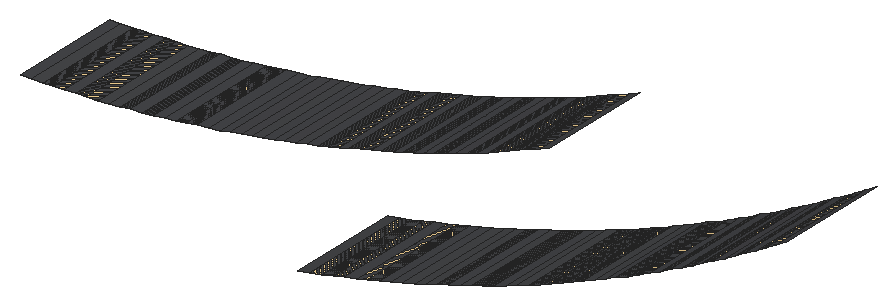
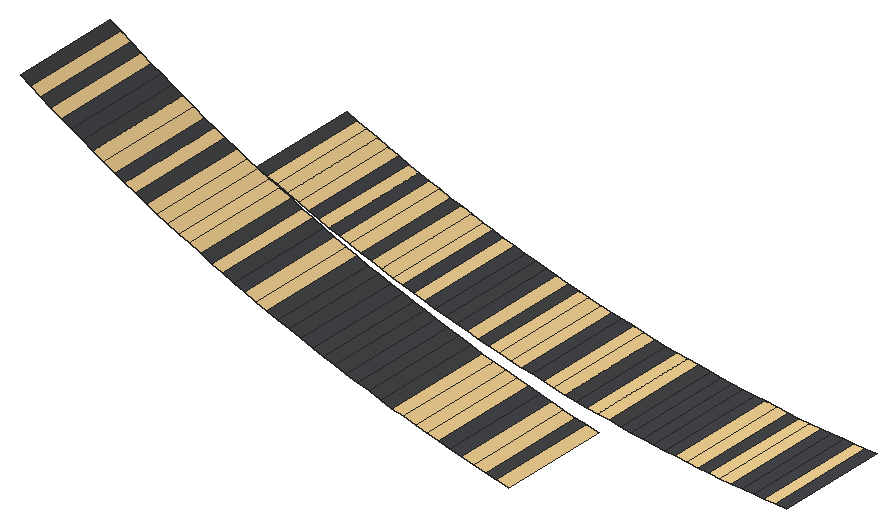
# SketchUp Ruby script. Lengths in inches.
U = 1.inch
M = Sketchup.active_model
def pt(a) = Geom::Point3d.new(a.map { |v| v * U })
def face(e, loops, mat)
  f = e.add_face(loops[0].map { |a| pt(a) })
  loops[1..].each { |l| e.add_face(l.map { |a| pt(a) }).erase! }
  f.material = f.back_material = mat if mat
  f
end
# faces: each face lists its corners as indices into pts; further lists are holes
def faces(e, pts, list, mat = nil) = list.each { |f| face(e, (f[0].is_a?(Array) ? f : [f]).map { |l| l.map { |i| pts[i] } }, mat) }
# xy, xz, yz: faces in a plane at the given z, y or x. An outline is a flat list of corners, or four numbers for a rectangle; further outlines are holes
def ring(l) = l.size == 4 ? [[l[0], l[1]], [l[2], l[1]], [l[2], l[3]], [l[0], l[3]]] : l.each_slice(2).to_a
def flat(e, list, mat, &to3) = list.each { |f| face(e, (f[0].is_a?(Array) ? f : [f]).map { |l| ring(l).map { |u, v| to3.(u, v) } }, mat) }
def xy(e, z, list, mat = nil) = flat(e, list, mat) { |x, y| [x, y, z] }
def xz(e, y, list, mat = nil) = flat(e, list, mat) { |x, z| [x, y, z] }
def yz(e, x, list, mat = nil) = flat(e, list, mat) { |y, z| [x, y, z] }
def lines(e, pts, list) = list.each { |a, b| e.add_line(pt(pts[a]), pt(pts[b])) }
# prism: a flat outline (further loops are holes) pulled along v
def prism(e, loops, v, mat = nil)
  f = face(e, loops, mat); d = Geom::Vector3d.new(v.map { |x| x * U })
  f.pushpull(f.normal.samedirection?(d) ? d.length : -d.length)
end
def box(e, o, s, mat = nil) = prism(e, [[o, [o[0] + s[0], o[1], o[2]], [o[0] + s[0], o[1] + s[1], o[2]], [o[0], o[1] + s[1], o[2]]]], [0, 0, s[2]], mat)
def at(x, y, z, deg = 0) = Geom::Transformation.translation(pt([x, y, z])) * Geom::Transformation.rotation(ORIGIN, Z_AXIS, deg.degrees)
def axes(o, x, y, z) = Geom::Transformation.new([*x, 0, *y, 0, *z, 0, *pt(o).to_a, 1])
def part(name) = M.definitions.add(name)
# library, detail: a bought-in or finely detailed component or shape, given as its bounding box
def library(name, o, s) = part(name).tap { |d| box(d.entities, o, s) }
def detail(e, o, s) = box(e.add_group.entities, o, s)
def put(e, d, t, mat = nil) = e.add_instance(d, t).tap { |i| i.material = mat if mat }
def group(e, t, mat = nil) = e.add_group.tap { |g| g.transformation = t; g.material = mat if mat }.entities
root = M.entities
M.materials.add("1432 AP 8245 TAR ROAD").color = [71, 72, 75]
M.materials.add("Outer Light").color = [251, 217, 152]
p = [[541.31,95.37,171.75],[541.47,95.37,171.79],[541.47,96.87,171.79],[541.31,96.87,171.75],[541.31,96.87,171.75],[541.47,96.87,171.79],
  [541.47,95.37,171.79],[541.31,95.37,171.75],[541.63,95.37,171.82],[541.63,96.87,171.82],[541.63,96.87,171.82],[541.63,95.37,171.82],
  [541.79,95.37,171.86],[541.79,96.87,171.86],[541.79,96.87,171.86],[541.79,95.37,171.86],[541.94,95.37,171.9],[541.94,96.87,171.9],
  [541.94,96.87,171.9],[541.94,95.37,171.9],[542.1,95.37,171.9375],[542.1,96.87,171.9375],[542.1,96.87,171.9375],[542.1,95.37,171.9375],
  [542.25,95.37,171.98],[542.25,96.87,171.98],[542.25,96.87,171.98],[542.25,95.37,171.98],[542.41,95.37,172.02],[542.41,96.87,172.02],
  [542.41,96.87,172.02],[542.41,95.37,172.02],[542.56,95.37,172.0625],[542.56,96.87,172.0625],[542.56,96.87,172.0625],[542.56,95.37,172.0625],
  [542.72,95.37,172.11],[542.72,96.87,172.11],[542.72,96.87,172.11],[542.72,95.37,172.11],[542.875,95.37,172.15],[542.875,96.87,172.15],
  [542.875,96.87,172.15],[542.875,95.37,172.15],[543.03,95.37,172.2],[543.03,96.87,172.2],[543.03,96.87,172.2],[543.03,95.37,172.2],
  [543.18,95.37,172.25],[543.18,96.87,172.25],[543.18,96.87,172.25],[543.18,95.37,172.25],[543.33,95.37,172.3],[543.33,96.87,172.3],
  [543.33,96.87,172.3],[543.33,95.37,172.3],[543.49,95.37,172.35],[543.49,96.87,172.35],[543.49,96.87,172.35],[543.49,95.37,172.35],
  [543.64,95.37,172.4],[543.64,96.87,172.4],[543.64,96.87,172.4],[543.64,95.37,172.4],[543.79,95.37,172.45],[543.79,96.87,172.45],
  [543.79,96.87,172.45],[543.79,95.37,172.45],[543.94,95.37,172.5],[543.94,96.87,172.5],[543.94,96.87,172.5],[543.94,95.37,172.5],
  [544.1,95.37,172.56],[544.1,96.87,172.56],[544.1,96.87,172.56],[544.1,95.37,172.56],[544.25,95.37,172.62],[544.25,96.87,172.62],
  [544.25,96.87,172.62],[544.25,95.37,172.62],[544.4,95.37,172.67],[544.4,96.87,172.67],[544.4,96.87,172.67],[544.4,95.37,172.67],
  [544.55,95.37,172.73],[544.55,96.87,172.73],[544.55,96.87,172.73],[544.55,95.37,172.73],[544.7,95.37,172.79],[544.7,96.87,172.79],
  [544.7,96.87,172.79],[544.7,95.37,172.79],[537.75,95.37,172.81],[537.6,95.37,172.8],[537.6,96.87,172.8],[537.75,96.87,172.81],
  [537.75,96.87,172.81],[537.6,96.87,172.8],[537.6,95.37,172.8],[537.75,95.37,172.81],[537.9,95.37,172.8125],[537.9,96.87,172.8125],
  [537.9,96.87,172.8125],[537.9,95.37,172.8125],[538.04,95.37,172.82],[538.04,96.87,172.82],[538.04,96.87,172.82],[538.04,95.37,172.82],
  [538.19,95.37,172.83],[538.19,96.87,172.83],[538.19,96.87,172.83],[538.19,95.37,172.83],[538.34,95.37,172.84],[538.34,96.87,172.84],
  [538.34,96.87,172.84],[538.34,95.37,172.84],[538.49,95.37,172.85],[538.49,96.87,172.85],[538.49,96.87,172.85],[538.49,95.37,172.85],
  [544.85,95.37,172.85],[544.85,96.87,172.85],[544.85,96.87,172.85],[544.85,95.37,172.85],[538.64,95.37,172.86],[538.64,96.87,172.86],
  [538.64,96.87,172.86],[538.64,95.37,172.86],[538.79,95.37,172.875],[538.79,96.87,172.875],[538.79,96.87,172.875],[538.79,95.37,172.875],
  [538.9375,95.37,172.89],[538.9375,96.87,172.89],[538.9375,96.87,172.89],[538.9375,95.37,172.89],[539.08,95.37,172.91],[539.08,96.87,172.91],
  [539.08,96.87,172.91],[539.08,95.37,172.91],[539.23,95.37,172.92],[539.23,96.87,172.92],[539.23,96.87,172.92],[539.23,95.37,172.92],
  [539.38,95.37,172.94],[539.38,96.87,172.94],[539.38,96.87,172.94],[539.38,95.37,172.94],[539.53,95.37,172.96],[539.53,96.87,172.96],
  [539.53,96.87,172.96],[539.53,95.37,172.96],[544.99,95.37,172.91],[544.99,96.87,172.91],[544.99,96.87,172.91],[544.99,95.37,172.91],
  [545.14,95.37,172.98],[545.14,96.87,172.98],[545.14,96.87,172.98],[545.14,95.37,172.98],[539.68,95.37,172.98],[539.68,96.87,172.98],
  [539.68,96.87,172.98],[539.68,95.37,172.98],[539.82,95.37,173],[539.82,96.87,173],[539.82,96.87,173],[539.82,95.37,173],
  [539.97,95.37,173.03],[539.97,96.87,173.03],[539.97,96.87,173.03],[539.97,95.37,173.03],[540.12,95.37,173.05],[540.12,96.87,173.05],
  [540.12,96.87,173.05],[540.12,95.37,173.05],[540.27,95.37,173.07],[540.27,96.87,173.07],[540.27,96.87,173.07],[540.27,95.37,173.07],
  [545.29,95.37,173.04],[545.29,96.87,173.04],[545.29,96.87,173.04],[545.29,95.37,173.04],[545.4375,95.37,173.11],[545.4375,96.87,173.11],
  [545.4375,96.87,173.11],[545.4375,95.37,173.11],[540.41,95.37,173.1],[540.41,96.87,173.1],[540.41,96.87,173.1],[540.41,95.37,173.1],
  [540.56,95.37,173.13],[540.56,96.87,173.13],[540.56,96.87,173.13],[540.56,95.37,173.13],[540.71,95.37,173.16],[540.71,96.87,173.16],
  [540.71,96.87,173.16],[540.71,95.37,173.16],[545.58,95.37,173.18],[545.58,96.87,173.18],[545.58,96.87,173.18],[545.58,95.37,173.18],
  [540.85,95.37,173.1875],[540.85,96.87,173.1875],[540.85,96.87,173.1875],[540.85,95.37,173.1875],[541,95.37,173.22],[541,96.87,173.22],
  [541,96.87,173.22],[541,95.37,173.22],[541.14,95.37,173.25],[541.14,96.87,173.25],[541.14,96.87,173.25],[541.14,95.37,173.25],
  [541.29,95.37,173.28],[541.29,96.87,173.28],[541.29,96.87,173.28],[541.29,95.37,173.28],[545.73,95.37,173.24],[545.73,96.87,173.24],
  [545.73,96.87,173.24],[545.73,95.37,173.24],[545.875,95.37,173.3125],[545.875,96.87,173.3125],[545.875,96.87,173.3125],[545.875,95.37,173.3125],
  [541.44,95.37,173.32],[541.44,96.87,173.32],[541.44,96.87,173.32],[541.44,95.37,173.32],[541.58,95.37,173.35],[541.58,96.87,173.35],
  [541.58,96.87,173.35],[541.58,95.37,173.35],[546.02,95.37,173.38],[546.02,96.87,173.38],[546.02,96.87,173.38],[546.02,95.37,173.38],
  [541.73,95.37,173.39],[541.73,96.87,173.39],[541.73,96.87,173.39],[541.73,95.37,173.39],[541.87,95.37,173.43],[541.87,96.87,173.43],
  [541.87,96.87,173.43],[541.87,95.37,173.43],[542.01,95.37,173.47],[542.01,96.87,173.47],[542.01,96.87,173.47],[542.01,95.37,173.47],
  [546.16,95.37,173.45],[546.16,96.87,173.45],[546.16,96.87,173.45],[546.16,95.37,173.45],[542.16,95.37,173.51],[542.16,96.87,173.51],
  [542.16,96.87,173.51],[542.16,95.37,173.51],[542.3,95.37,173.55],[542.3,96.87,173.55],[542.3,96.87,173.55],[542.3,95.37,173.55],
  [542.44,95.37,173.59],[542.44,96.87,173.59],[542.44,96.87,173.59],[542.44,95.37,173.59],[546.31,95.37,173.53],[546.31,96.87,173.53],
  [546.31,96.87,173.53],[546.31,95.37,173.53],[546.45,95.37,173.6],[546.45,96.87,173.6],[546.45,96.87,173.6],[546.45,95.37,173.6],
  [542.59,95.37,173.63],[542.59,96.87,173.63],[542.59,96.87,173.63],[542.59,95.37,173.63],[542.73,95.37,173.68],[542.73,96.87,173.68],
  [542.73,96.87,173.68],[542.73,95.37,173.68],[546.59,95.37,173.67],[546.59,96.87,173.67],[546.59,96.87,173.67],[546.59,95.37,173.67],
  [542.87,95.37,173.72],[542.87,96.87,173.72],[542.87,96.87,173.72],[542.87,95.37,173.72],[543.01,95.37,173.77],[543.01,96.87,173.77],
  [543.01,96.87,173.77],[543.01,95.37,173.77],[546.73,95.37,173.75],[546.73,96.87,173.75],[546.73,96.87,173.75],[546.73,95.37,173.75],
  [543.15,95.37,173.82],[543.15,96.87,173.82],[543.15,96.87,173.82],[543.15,95.37,173.82],[543.3,95.37,173.87],[543.3,96.87,173.87],
  [543.3,96.87,173.87],[543.3,95.37,173.87],[546.875,95.37,173.83],[546.875,96.87,173.83],[546.875,96.87,173.83],[546.875,95.37,173.83],
  [547.02,95.37,173.91],[547.02,96.87,173.91],[547.02,96.87,173.91],[547.02,95.37,173.91],[543.4375,95.37,173.92],[543.4375,96.87,173.92],
  [543.4375,96.87,173.92],[543.4375,95.37,173.92],[543.58,95.37,173.97],[543.58,96.87,173.97],[543.58,96.87,173.97],[543.58,95.37,173.97],
  [547.16,95.37,173.99],[547.16,96.87,173.99],[547.16,96.87,173.99],[547.16,95.37,173.99],[543.72,95.37,174.02],[543.72,96.87,174.02],
  [543.72,96.87,174.02],[543.72,95.37,174.02],[543.86,95.37,174.07],[543.86,96.87,174.07],[543.86,96.87,174.07],[543.86,95.37,174.07],
  [547.3,95.37,174.07],[547.3,96.87,174.07],[547.3,96.87,174.07],[547.3,95.37,174.07],[543.99,95.37,174.125],[543.99,96.87,174.125],
  [543.99,96.87,174.125],[543.99,95.37,174.125],[544.13,95.37,174.18],[544.13,96.87,174.18],[544.13,96.87,174.18],[544.13,95.37,174.18],
  [547.44,95.37,174.15],[547.44,96.87,174.15],[547.44,96.87,174.15],[547.44,95.37,174.15],[547.57,95.37,174.23],[547.57,96.87,174.23],
  [547.57,96.87,174.23],[547.57,95.37,174.23],[544.27,95.37,174.24],[544.27,96.87,174.24],[544.27,96.87,174.24],[544.27,95.37,174.24],
  [544.41,95.37,174.3],[544.41,96.87,174.3],[544.41,96.87,174.3],[544.41,95.37,174.3],[547.71,95.37,174.3125],[547.71,96.87,174.3125],
  [547.71,96.87,174.3125],[547.71,95.37,174.3125],[544.55,95.37,174.35],[544.55,96.87,174.35],[544.55,96.87,174.35],[544.55,95.37,174.35],
  [547.85,95.37,174.4],[547.85,96.87,174.4],[547.85,96.87,174.4],[547.85,95.37,174.4],[544.68,95.37,174.41],[544.68,96.87,174.41]]
faces(root,p,[[0,1,2,3],[1,8,9,2],[8,12,13,9],[12,16,17,13],[16,20,21,17],[20,24,25,21],[24,28,29,25],[28,32,33,29],
  [32,36,37,33],[36,40,41,37],[40,44,45,41],[44,48,49,45],[48,52,53,49],[52,56,57,53],[56,60,61,57],[60,64,65,61],
  [64,68,69,65],[68,72,73,69],[72,76,77,73],[76,80,81,77],[80,84,85,81],[84,88,89,85],[92,93,94,95],[100,92,95,101],
  [104,100,101,105],[108,104,105,109],[112,108,109,113],[116,112,113,117],[88,120,121,89],[124,116,117,125],[128,124,125,129],[132,128,129,133],
  [136,132,133,137],[140,136,137,141],[144,140,141,145],[148,144,145,149],[120,152,153,121],[152,156,157,153],[160,148,149,161],[164,160,161,165],
  [168,164,165,169],[172,168,169,173],[176,172,173,177],[156,180,181,157],[180,184,185,181],[188,176,177,189],[192,188,189,193],[196,192,193,197],
  [184,200,201,185],[204,196,197,205],[208,204,205,209],[212,208,209,213],[216,212,213,217],[200,220,221,201],[220,224,225,221],[228,216,217,229],
  [232,228,229,233],[224,236,237,225],[240,232,233,241],[244,240,241,245],[248,244,245,249],[236,252,253,237],[256,248,249,257],[260,256,257,261],
  [264,260,261,265],[252,268,269,253],[268,272,273,269],[276,264,265,277],[280,276,277,281],[272,284,285,273],[288,280,281,289],[292,288,289,293],
  [284,296,297,285],[300,292,293,301],[304,300,301,305],[296,308,309,297],[308,312,313,309],[316,304,305,317],[320,316,317,321],[312,324,325,313],
  [328,320,321,329],[332,328,329,333],[324,336,337,325],[340,332,333,341],[344,340,341,345],[336,348,349,337],[348,352,353,349],[356,344,345,357],
  [360,356,357,361],[352,364,365,353],[368,360,361,369],[364,372,373,365],[376,368,369,377]],"1432 AP 8245 TAR ROAD")
faces(root,p,[[4,5,6,7],[5,10,11,6],[10,14,15,11],[14,18,19,15],[18,22,23,19],[22,26,27,23],[26,30,31,27],[30,34,35,31],
  [34,38,39,35],[38,42,43,39],[42,46,47,43],[46,50,51,47],[50,54,55,51],[54,58,59,55],[58,62,63,59],[62,66,67,63],
  [66,70,71,67],[70,74,75,71],[74,78,79,75],[78,82,83,79],[82,86,87,83],[86,90,91,87],[96,97,98,99],[102,96,99,103],
  [106,102,103,107],[110,106,107,111],[114,110,111,115],[118,114,115,119],[90,122,123,91],[126,118,119,127],[130,126,127,131],[134,130,131,135],
  [138,134,135,139],[142,138,139,143],[146,142,143,147],[150,146,147,151],[122,154,155,123],[154,158,159,155],[162,150,151,163],[166,162,163,167],
  [170,166,167,171],[174,170,171,175],[178,174,175,179],[158,182,183,159],[182,186,187,183],[190,178,179,191],[194,190,191,195],[198,194,195,199],
  [186,202,203,187],[206,198,199,207],[210,206,207,211],[214,210,211,215],[218,214,215,219],[202,222,223,203],[222,226,227,223],[230,218,219,231],
  [234,230,231,235],[226,238,239,227],[242,234,235,243],[246,242,243,247],[250,246,247,251],[238,254,255,239],[258,250,251,259],[262,258,259,263],
  [266,262,263,267],[254,270,271,255],[270,274,275,271],[278,266,267,279],[282,278,279,283],[274,286,287,275],[290,282,283,291],[294,290,291,295],
  [286,298,299,287],[302,294,295,303],[306,302,303,307],[298,310,311,299],[310,314,315,311],[318,306,307,319],[322,318,319,323],[314,326,327,315],
  [330,322,323,331],[334,330,331,335],[326,338,339,327],[342,334,335,343],[346,342,343,347],[338,350,351,339],[350,354,355,351],[358,346,347,359],
  [362,358,359,363],[354,366,367,355],[370,362,363,371],[366,374,375,367]],"Outer Light")
